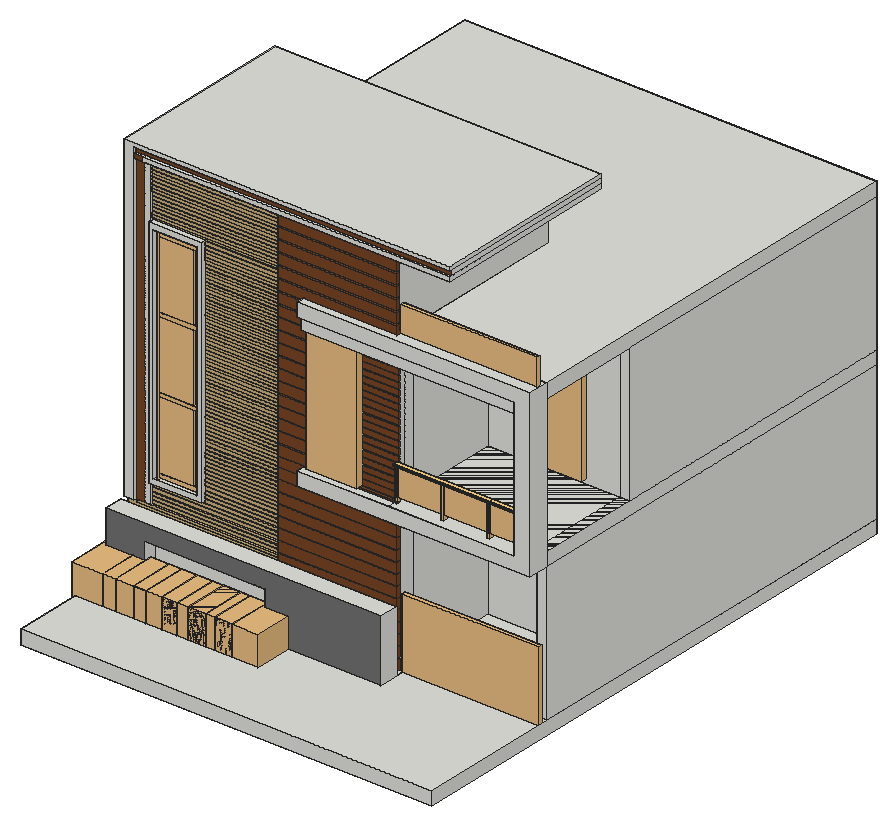
# SketchUp Ruby script. Lengths in inches.
U = 1.inch
M = Sketchup.active_model
def pt(a) = Geom::Point3d.new(a.map { |v| v * U })
def face(e, loops, mat)
  f = e.add_face(loops[0].map { |a| pt(a) })
  loops[1..].each { |l| e.add_face(l.map { |a| pt(a) }).erase! }
  f.material = f.back_material = mat if mat
  f
end
# faces: each face lists its corners as indices into pts; further lists are holes
def faces(e, pts, list, mat = nil) = list.each { |f| face(e, (f[0].is_a?(Array) ? f : [f]).map { |l| l.map { |i| pts[i] } }, mat) }
# xy, xz, yz: faces in a plane at the given z, y or x. An outline is a flat list of corners, or four numbers for a rectangle; further outlines are holes
def ring(l) = l.size == 4 ? [[l[0], l[1]], [l[2], l[1]], [l[2], l[3]], [l[0], l[3]]] : l.each_slice(2).to_a
def flat(e, list, mat, &to3) = list.each { |f| face(e, (f[0].is_a?(Array) ? f : [f]).map { |l| ring(l).map { |u, v| to3.(u, v) } }, mat) }
def xy(e, z, list, mat = nil) = flat(e, list, mat) { |x, y| [x, y, z] }
def xz(e, y, list, mat = nil) = flat(e, list, mat) { |x, z| [x, y, z] }
def yz(e, x, list, mat = nil) = flat(e, list, mat) { |y, z| [x, y, z] }
def lines(e, pts, list) = list.each { |a, b| e.add_line(pt(pts[a]), pt(pts[b])) }
# prism: a flat outline (further loops are holes) pulled along v
def prism(e, loops, v, mat = nil)
  f = face(e, loops, mat); d = Geom::Vector3d.new(v.map { |x| x * U })
  f.pushpull(f.normal.samedirection?(d) ? d.length : -d.length)
end
def box(e, o, s, mat = nil) = prism(e, [[o, [o[0] + s[0], o[1], o[2]], [o[0] + s[0], o[1] + s[1], o[2]], [o[0], o[1] + s[1], o[2]]]], [0, 0, s[2]], mat)
def at(x, y, z, deg = 0) = Geom::Transformation.translation(pt([x, y, z])) * Geom::Transformation.rotation(ORIGIN, Z_AXIS, deg.degrees)
def axes(o, x, y, z) = Geom::Transformation.new([*x, 0, *y, 0, *z, 0, *pt(o).to_a, 1])
def part(name) = M.definitions.add(name)
# library, detail: a bought-in or finely detailed component or shape, given as its bounding box
def library(name, o, s) = part(name).tap { |d| box(d.entities, o, s) }
def detail(e, o, s) = box(e.add_group.entities, o, s)
def put(e, d, t, mat = nil) = e.add_instance(d, t).tap { |i| i.material = mat if mat }
def group(e, t, mat = nil) = e.add_group.tap { |g| g.transformation = t; g.material = mat if mat }.entities
root = M.entities
M.materials.add("4wer gsdf uhghh1").color = [251, 209, 129]
M.materials.add("[0128_White]").color = [255, 255, 255]
M.materials.add("[0130_Gainsboro]").color = [220, 220, 220]
M.materials.add("[Color M05]").color = [114, 114, 114]
M.materials.add("[Wood Floor Light]").color = [204, 176, 127]
M.materials.add("[Wood Veneer 01]").color = [120, 70, 37]
c1 = library("CNC CUTTING TEXTURE",[0,0,-0.79],[85.98,295.47,0.79])
c2 = library("Untitled",[0,0,0],[36,4.39,84])
c3 = library("GATE DESIGN",[0,0,0],[157.48,1.97,82.05])
c4 = library("Raiing",[0,0,0],[2.36,157.48,43.31])
c5 = library("Line03",[-161.9,-1.5,-0.01],[5.61,3,76.05])
c6 = library("Rectangle2",[-158.32,-0.85,10.07],[105.83,1.72,65.72])
c7 = part("Rectangle3")
prism(c7.entities,[[[162.42,-2.78,77.23],[162.42,-2.8125,75.23],[162.42,2.82,75.23],[162.42,2.79,77.23],[162.42,2.57,77.68],[162.42,2.18,77.99],[162.42,1.69,78.1],[162.42,-1.68,78.1],[162.42,-2.17,77.99],[162.42,-2.5625,77.68]]],[-327.5,0,0],"4wer gsdf uhghh1")
c8 = part("skp26F")
put(c8.entities,c5,at(0,0,0))
put(c8.entities,c6,at(0,0,0))
put(c8.entities,c7,at(0,0,0))
put(c8.entities,c5,at(105.79,0,0))
put(c8.entities,c6,at(105.79,0,0))
put(c8.entities,c6,at(211.06,0,0))
put(c8.entities,c5,at(211.06,0,0))
put(c8.entities,c5,at(316.15,0,0))
c9 = part("Railing1")
put(c9.entities,c8,at(161.9,1.5,0.01))
c10 = part("plafonjera 30x30")
g1 = group(c10.entities,at(0,49.12,61.9),"[0128_White]")
xy(g1,-1.18,[[[0,-11.8125,11.8125,0],[0.79,-11.02,11.02,-0.79]]],"[0130_Gainsboro]")
xy(g1,-0.98,[[0.79,-11.02,11.02,-0.79]],"[0128_White]")
xy(g1,0,[[0,-11.8125,11.8125,0]],"[0130_Gainsboro]")
xz(g1,-11.8125,[[0,-1.18,11.8125,0]],"[0130_Gainsboro]")
xz(g1,-11.02,[[0.79,-1.18,11.02,-0.98]],"[0130_Gainsboro]")
xz(g1,-0.79,[[0.79,-1.18,11.02,-0.98]],"[0130_Gainsboro]")
xz(g1,0,[[0,-1.18,11.8125,0]],"[0130_Gainsboro]")
yz(g1,0,[[-11.8125,-1.18,0,0]],"[0130_Gainsboro]")
yz(g1,0.79,[[-11.02,-1.18,-0.79,-0.98]],"[0130_Gainsboro]")
yz(g1,11.02,[[-11.02,-1.18,-0.79,-0.98]],"[0130_Gainsboro]")
yz(g1,11.8125,[[-11.8125,-1.18,0,0]],"[0130_Gainsboro]")
c11 = library("planta",[-33.71,-17.92,-17.375],[61.06,56.98,83.04])
c12 = part("Group\#3")
box(c12.entities,[0,-0.9375,0],[32.21,0.9375,4.8125])
c13 = part("Group\#6")
box(c13.entities,[0,-3.3125,0],[104.3,3.3125,9.03])
c14 = part("Group\#5")
box(c14.entities,[78.86,-3.3125,0],[25.44,3.3125,9.03])
c15 = part("Group\#8")
box(c15.entities,[0,-1.625,0],[111.71,1.625,2.46])
c16 = part("Group\#14")
box(c16.entities,[108.55,-1.625,58.72],[65.17,1.625,2.46])
xy(root,-12,[[2.57,92.9375,2.57,125.4375,158.82,125.4375,158.82,117.5,243.57,117.5,243.57,92.9375]])
xy(root,-2.01,[[36.8125,92.9375,141.8125,104.3125]])
xy(root,0,[[2.57,109.79,243.57,117.5],[[158.82,117.5,238.63,117.5,238.63,215.88,353.57,215.88,353.57,125.4375,362.57,125.4375,362.57,485.4375,2.57,485.4375,2.57,125.4375,158.82,125.4375],[11.57,134.4375,11.57,476.4375,353.57,476.4375,353.57,224.88,229.63,224.88,229.63,134.4375]],[238.63,125.4375,353.57,134.4375],[11.57,134.4375,229.63,134.4375,229.63,224.88,353.57,224.88,353.57,476.4375,11.57,476.4375],[238.63,134.4375,353.57,215.88]])
xy(root,39.99,[[36.8125,92.9375,141.8125,104.3125]])
xy(root,54.0625,[[2.57,92.9375,243.57,109.79]])
xy(root,54.8125,[[2.57,113.25,11.57,117.5],[11.57,115.3125,18.82,117.5],[18.82,115.3125,24.75,117.5]])
xy(root,73.23,[[24.75,112.3125,71.07,117.5]])
xy(root,77.43,[[28.95,112.3125,66.875,117.5]])
xy(root,120,[[158.82,107.25,238.63,117.5],[238.63,107.25,362.57,125.4375],[158.82,117.5,238.63,125.4375],[[2.57,125.4375,238.63,125.4375,238.63,215.88,353.57,215.88,353.57,125.4375,362.57,125.4375,362.57,485.4375,2.57,485.4375],[11.57,134.4375,11.57,476.4375,353.57,476.4375,353.57,224.88,229.63,224.88,229.63,134.4375]]])
xy(root,132,[[158.82,107.25,238.63,107.25,238.63,119.75,206.42,119.75,206.42,117.5,158.82,117.5],[238.63,107.25,348.21,125.4375],[158.82,117.5,206.42,125.4375],[206.42,119.75,238.63,125.4375],[[2.57,125.4375,238.63,125.4375,238.63,215.88,362.57,215.88,362.57,485.4375,2.57,485.4375],[11.57,134.4375,11.57,476.4375,353.57,476.4375,353.57,224.88,229.63,224.88,229.63,134.4375]],
  [238.63,125.4375,362.57,125.4375,362.57,215.88,353.57,215.88,353.57,134.4375,238.63,134.4375],[11.57,134.4375,229.63,134.4375,229.63,224.88,353.57,224.88,353.57,476.4375,11.57,476.4375],[238.63,134.4375,353.57,215.88]])
xy(root,240.0625,[[158.82,111.375,158.82,117.5,206.42,117.5,206.42,119.75,238.63,119.75,238.63,125.4375,348.21,125.4375,348.21,111.375],[206.42,119.75,238.63,125.4375],[238.63,125.4375,348.21,134.4375]])
xy(root,252,[[158.82,107.25,348.21,111.375],[158.82,111.375,348.21,125.4375],[158.82,125.4375,348.21,125.4375,348.21,134.4375,238.63,134.4375,238.63,215.88,362.57,215.88,362.57,485.4375,2.57,485.4375,2.57,278.5625,11.57,278.5625,11.57,476.4375,353.57,476.4375,353.57,224.88,229.63,224.88,229.63,134.4375,158.82,134.4375],[2.57,125.4375,158.82,125.4375,158.82,134.4375,11.57,134.4375,11.57,278.5625,2.57,278.5625],[11.57,134.4375,158.82,278.5625]])
xy(root,264,[[158.82,107.25,362.57,107.25,362.57,125.4375,240.76,125.4375,240.76,117.5,158.82,117.5],[158.82,117.5,240.76,125.4375],[158.82,125.4375,240.76,278.5625]])
xy(root,272.98,[[28.95,112.3125,66.875,117.5]])
xy(root,277.17,[[24.75,112.3125,71.07,117.5]])
xy(root,322.4375,[[11.57,113.25,19.41,115.3125],[19.41,113.25,19.41,115.3125,24.75,115.3125,24.75,117.5,287.13,117.5,287.13,113.25],[11.57,117.5,18.82,125.4375],[18.82,117.5,24.75,278.5625],[24.75,117.5,240.76,278.5625],
  [240.76,117.5,287.13,278.5625],[11.57,125.4375,18.82,278.5625]])
xy(root,326.28,[[11.57,113.25,11.57,115.3125,18.82,115.3125,19.41,113.25],[19.41,113.25,18.82,115.3125,287.13,115.3125,287.13,113.25],[24.75,115.3125,287.13,278.5625]])
xy(root,330.84,[[11.57,113.25,18.82,115.3125],[18.82,113.25,287.13,115.3125],[11.57,115.3125,18.82,125.4375],[18.82,115.3125,287.13,278.5625],[11.57,125.4375,18.82,278.5625]])
xy(root,334.25,[[2.57,113.25,287.13,278.5625]])
xz(root,92.9375,[[[2.57,-12,243.57,54.0625],[36.8125,-2.01,141.8125,39.99]]],"[Color M05]")
xz(root,104.3125,[[36.8125,-2.01,141.8125,39.99]])
xz(root,107.25,[[158.82,120,362.57,120,362.57,264,158.82,264,158.82,252,348.21,252,348.21,132,158.82,132]])
xz(root,109.79,[[2.57,0,243.57,54.0625]])
xz(root,111.375,[[158.82,240.0625,348.21,252]])
xz(root,112.3125,[[[24.75,73.23,71.07,277.17],[28.95,77.43,66.875,272.98]]])
xz(root,113.25,[[2.57,54.8125,11.57,54.8125,11.57,330.84,287.13,330.84,287.13,334.25,2.57,334.25],[19.41,322.4375,287.13,326.28]])
xz(root,113.25,[[11.57,322.4375,19.41,326.28]],"[Wood Veneer 01]")
xz(root,115.3125,[[18.82,54.8125,24.75,322.4375],[11.57,322.4375,24.75,326.28]])
xz(root,115.3125,[[11.57,54.8125,18.82,322.4375],[11.57,326.28,18.82,330.84],[18.82,326.28,287.13,330.84]],"[Wood Veneer 01]")
xz(root,117.5,[[158.82,-12,243.57,0],[136.46,0,238.63,0,238.63,120,158.82,120,158.82,132,206.42,132,206.42,240.0625,158.82,240.0625,158.82,264,240.76,264,240.76,313.41,136.46,313.41],[11.57,54.8125,18.82,322.4375],[18.82,54.8125,24.75,322.4375],[28.95,77.43,66.875,272.98]])
xz(root,117.5,[[2.57,0,136.46,0,136.46,319.98,24.75,319.98,24.75,277.17,71.07,277.17,71.07,73.23,24.75,73.23,24.75,54.8125,2.57,54.8125]],"[Wood Floor Light]")
xz(root,119.75,[[206.42,132,238.63,235.25]],"[Wood Veneer 01]")
xz(root,125.4375,[[2.57,-12,158.82,0],[2.57,0,158.82,120],[353.57,0,362.57,120],[2.57,120,158.82,132],[158.82,120,362.57,132],
  [2.57,132,158.82,252],[348.21,132,348.21,252,158.82,252,158.82,264,362.57,264,362.57,132],[206.42,132,238.63,240.0625],[11.57,322.4375,18.82,330.84]])
xz(root,134.4375,[[11.57,0,229.63,120],[11.57,132,229.63,252],[238.63,240.0625,348.21,252]])
xz(root,215.88,[[238.63,0,353.57,120],[238.63,132,353.57,252],[353.57,132,362.57,252]])
xz(root,224.88,[[229.63,0,353.57,120],[229.63,132,353.57,252]])
xz(root,278.5625,[[2.57,252,158.82,252,158.82,264,240.76,264,240.76,322.4375,11.57,322.4375,11.57,330.84,287.13,330.84,287.13,334.25,2.57,334.25],[18.82,322.4375,18.82,330.84,287.13,330.84,287.13,326.28,24.75,326.28,24.75,322.4375],[24.75,322.4375,287.13,326.28]])
xz(root,476.4375,[[11.57,0,353.57,120],[11.57,132,353.57,252]])
xz(root,485.4375,[[2.57,0,362.57,120],[2.57,132,362.57,252]])
yz(root,2.57,[[92.9375,-12,92.9375,54.0625,109.79,54.0625,109.79,0,117.5,0,117.5,54.8125,113.25,54.8125,113.25,334.25,278.5625,334.25,278.5625,252,125.4375,252,125.4375,-12],[125.4375,0,485.4375,120],[125.4375,132,485.4375,252]])
yz(root,11.57,[[134.4375,0,476.4375,120],[113.25,54.8125,115.3125,322.4375],[115.3125,54.8125,115.3125,330.84,125.4375,330.84,125.4375,322.4375,117.5,322.4375,117.5,54.8125],[134.4375,132,476.4375,252],[113.25,322.4375,115.3125,326.28],
  [125.4375,322.4375,278.5625,330.84],[113.25,326.28,115.3125,330.84]])
yz(root,18.82,[[125.4375,322.4375,278.5625,330.84]])
yz(root,24.75,[[115.3125,54.8125,117.5,73.23],[112.3125,73.23,115.3125,277.17],[115.3125,73.23,117.5,277.17],[115.3125,277.17,117.5,322.4375],[115.3125,322.4375,278.5625,326.28]])
yz(root,28.95,[[112.3125,77.43,117.5,272.98]])
yz(root,36.8125,[[92.9375,-2.01,104.3125,39.99]])
yz(root,66.875,[[112.3125,77.43,117.5,272.98]])
yz(root,71.07,[[112.3125,73.23,117.5,277.17]])
yz(root,141.8125,[[92.9375,-2.01,104.3125,39.99]])
yz(root,158.82,[[117.5,-12,125.4375,0],[107.25,120,117.5,132],[117.5,120,125.4375,132],[111.375,240.0625,117.5,252],[117.5,240.0625,125.4375,252],
  [107.25,252,117.5,264],[117.5,252,125.4375,264],[125.4375,252,278.5625,264]])
yz(root,206.42,[[117.5,132,119.75,240.0625],[119.75,132,125.4375,240.0625]])
yz(root,229.63,[[134.4375,0,224.88,120],[134.4375,132,224.88,252]])
yz(root,238.63,[[117.5,0,134.4375,120],[134.4375,0,215.88,120],[119.75,132,125.4375,240.0625],[125.4375,132,134.4375,240.0625],[134.4375,132,215.88,252]])
yz(root,240.76,[[117.5,264,278.5625,322.4375]])
yz(root,243.57,[[92.9375,-12,117.5,-12,117.5,0,109.79,0,109.79,54.0625,92.9375,54.0625]])
yz(root,287.13,[[113.25,322.4375,278.5625,326.28],[115.3125,326.28,278.5625,330.84],[113.25,330.84,278.5625,334.25]])
yz(root,348.21,[[107.25,132,107.25,252,111.375,252,111.375,240.0625,125.4375,240.0625,125.4375,132],[111.375,240.0625,125.4375,252],[125.4375,240.0625,134.4375,252]])
yz(root,353.57,[[125.4375,0,215.88,120],[224.88,0,476.4375,120],[224.88,132,476.4375,252]])
yz(root,362.57,[[125.4375,0,485.4375,120],[107.25,120,125.4375,264],[215.88,132,485.4375,252]])
put(root,c1,axes([161.91,121.89,132],[0.51768,0,0],[0,0,0.36573],[0,11.28983,0]))
put(root,c2,at(288.11,211.49,135.42))
put(root,c2,at(288.11,211.49,4.48))
put(root,c3,axes([243.57,116.18,0],[0.7556,0,0],[0,1.67,0],[0,0,0.75]))
put(root,c4,axes([240.76,119.86,258.57],[0,-1,0],[0.76,0,0],[0,0,0.66]))
put(root,c9,axes([238.79,114.1875,132.875],[0.38166,0,0],[0,1,0],[0,0,0.37]))
put(root,c10,at(264.84,88.8125,259.79))
put(root,c10,at(264.84,126.125,259.79))
put(root,c10,at(264.84,163.1875,259.79))
put(root,c10,at(264.84,197.8125,259.79))
put(root,c9,axes([66.67,114.1875,79.33],[0,0,0.5971],[0,1,0],[-0.4588,0,0]))
put(root,c11,axes([20.57,72.33,-7.52],[0.6248,0,0],[0,0.68,0],[0,0,0.50364]))
put(root,c11,axes([47.38,72.33,-7.52],[0.6248,0,0],[0,0.68,0],[0,0,0.50364]))
put(root,c11,axes([74.51,72.33,-7.52],[0.6248,0,0],[0,0.68,0],[0,0,0.50364]))
put(root,c11,axes([99.2,72.33,-7.52],[0.6248,0,0],[0,0.68,0],[0,0,0.50364]))
put(root,c11,axes([122.32,72.33,-7.52],[0.6248,0,0],[0,0.68,0],[0,0,0.50364]))
put(root,c11,axes([145.32,72.33,-7.52],[0.6248,0,0],[0,0.68,0],[0,0,0.50364]))
g2 = group(root,at(2.57,485.4375,-12))
box(g2,[0,-485.4375,0],[360,485.4375,12])
g3 = group(root,at(2.57,485.4375,120))
box(g3,[0,-360,0],[360,360,12])
g4 = group(root,at(2.57,485.4375,252))
box(g4,[0,-360,0],[360,360,12])
put(root,c12,at(206.42,119.75,235.25),"[Wood Veneer 01]")
put(root,c12,at(206.42,119.75,229.75),"[Wood Veneer 01]")
put(root,c12,at(206.42,119.75,224.375),"[Wood Veneer 01]")
put(root,c12,at(206.42,119.75,218.6875),"[Wood Veneer 01]")
put(root,c12,at(206.42,119.75,213.125),"[Wood Veneer 01]")
put(root,c12,at(206.42,119.75,207.375),"[Wood Veneer 01]")
put(root,c12,at(206.42,119.75,201.8125),"[Wood Veneer 01]")
put(root,c12,at(206.42,119.75,196.125),"[Wood Veneer 01]")
put(root,c12,at(206.42,119.75,190.3125),"[Wood Veneer 01]")
put(root,c12,at(206.42,119.75,184.1875),"[Wood Veneer 01]")
put(root,c12,at(206.42,119.75,178.5),"[Wood Veneer 01]")
put(root,c12,at(206.42,119.75,172.75),"[Wood Veneer 01]")
put(root,c12,at(206.42,119.75,167),"[Wood Veneer 01]")
put(root,c12,at(206.42,119.75,161.0625),"[Wood Veneer 01]")
put(root,c12,at(206.42,119.75,155),"[Wood Veneer 01]")
put(root,c12,at(206.42,119.75,149.4375),"[Wood Veneer 01]")
put(root,c12,at(206.42,119.75,143.5625),"[Wood Veneer 01]")
put(root,c12,at(206.42,119.75,137.8125),"[Wood Veneer 01]")
put(root,c12,at(206.42,119.75,132.3125),"[Wood Veneer 01]")
put(root,c13,at(136.46,117.5,313.41),"[Wood Veneer 01]")
put(root,c13,at(136.46,117.5,302.91),"[Wood Veneer 01]")
put(root,c13,at(136.46,117.5,292.84),"[Wood Veneer 01]")
put(root,c13,at(136.46,117.5,282.59),"[Wood Veneer 01]")
put(root,c13,at(136.46,117.5,272.53),"[Wood Veneer 01]")
put(root,c13,at(136.46,117.5,262.28),"[Wood Veneer 01]")
put(root,c13,at(136.46,117.5,252.22),"[Wood Veneer 01]")
put(root,c13,at(136.46,117.5,242.16),"[Wood Veneer 01]")
put(root,c14,at(57.6,117.5,232.09),"[Wood Veneer 01]")
put(root,c14,at(57.6,117.5,222.09),"[Wood Veneer 01]")
put(root,c14,at(57.6,117.5,212.09),"[Wood Veneer 01]")
put(root,c14,at(57.6,117.5,202.09),"[Wood Veneer 01]")
put(root,c14,at(57.6,117.5,192.22),"[Wood Veneer 01]")
put(root,c14,at(57.6,117.5,182.34),"[Wood Veneer 01]")
put(root,c14,at(57.6,117.5,172.47),"[Wood Veneer 01]")
put(root,c14,at(57.6,117.5,162.78),"[Wood Veneer 01]")
put(root,c14,at(57.6,117.5,152.97),"[Wood Veneer 01]")
put(root,c14,at(57.6,117.5,143.16),"[Wood Veneer 01]")
put(root,c14,at(57.6,117.5,132.59),"[Wood Veneer 01]")
put(root,c13,at(136.46,117.5,0),"[Wood Veneer 01]")
put(root,c13,at(136.46,117.5,9.9375),"[Wood Veneer 01]")
put(root,c13,at(136.46,117.5,19.5),"[Wood Veneer 01]")
put(root,c13,at(136.46,117.5,28.9375),"[Wood Veneer 01]")
put(root,c13,at(136.46,117.5,38.5),"[Wood Veneer 01]")
put(root,c13,at(136.46,117.5,47.9375),"[Wood Veneer 01]")
put(root,c13,at(136.46,117.5,57.5),"[Wood Veneer 01]")
put(root,c13,at(136.46,117.5,67.0625),"[Wood Veneer 01]")
put(root,c13,at(136.46,117.5,76.625),"[Wood Veneer 01]")
put(root,c13,at(136.46,117.5,86.125),"[Wood Veneer 01]")
put(root,c13,at(136.46,117.5,95.625),"[Wood Veneer 01]")
put(root,c13,at(136.46,117.5,105.25),"[Wood Veneer 01]")
put(root,c13,at(136.46,117.5,114.8125),"[Wood Veneer 01]")
put(root,c13,at(136.46,117.5,123.84),"[Wood Veneer 01]")
put(root,c15,at(24.75,117.5,319.98),"[Wood Floor Light]")
put(root,c15,at(24.75,117.5,317.16),"[Wood Floor Light]")
put(root,c15,at(24.75,117.5,314.35),"[Wood Floor Light]")
put(root,c15,at(24.75,117.5,311.54),"[Wood Floor Light]")
put(root,c15,at(24.75,117.5,308.6),"[Wood Floor Light]")
put(root,c15,at(24.75,117.5,305.66),"[Wood Floor Light]")
put(root,c15,at(24.75,117.5,302.73),"[Wood Floor Light]")
put(root,c15,at(24.75,117.5,299.79),"[Wood Floor Light]")
put(root,c15,at(24.75,117.5,296.91),"[Wood Floor Light]")
put(root,c15,at(24.75,117.5,293.91),"[Wood Floor Light]")
put(root,c15,at(24.75,117.5,290.98),"[Wood Floor Light]")
put(root,c15,at(24.75,117.5,288.1),"[Wood Floor Light]")
put(root,c15,at(24.75,117.5,285.16),"[Wood Floor Light]")
put(root,c15,at(24.75,117.5,282.35),"[Wood Floor Light]")
put(root,c15,at(24.75,117.5,279.54),"[Wood Floor Light]")
put(root,c16,at(-37.25,117.5,215.84),"[Wood Floor Light]")
put(root,c16,at(-37.25,117.5,212.02),"[Wood Floor Light]")
put(root,c16,at(-37.25,117.5,209.21),"[Wood Floor Light]")
put(root,c16,at(-37.25,117.5,206.4),"[Wood Floor Light]")
put(root,c16,at(-37.25,117.5,203.59),"[Wood Floor Light]")
put(root,c16,at(-37.48,117.5,200.89),"[Wood Floor Light]")
put(root,c16,at(-37.48,117.5,198.21),"[Wood Floor Light]")
put(root,c16,at(-37.48,117.5,195.27),"[Wood Floor Light]")
put(root,c16,at(-37.48,117.5,192.64),"[Wood Floor Light]")
put(root,c16,at(-37.48,117.5,189.89),"[Wood Floor Light]")
put(root,c16,at(-37.48,117.5,187.07),"[Wood Floor Light]")
put(root,c16,at(-37.48,117.5,184.32),"[Wood Floor Light]")
put(root,c16,at(-37.48,117.5,181.5),"[Wood Floor Light]")
put(root,c16,at(-37.48,117.5,178.93),"[Wood Floor Light]")
put(root,c16,at(-37.48,117.5,176.24),"[Wood Floor Light]")
put(root,c16,at(-37.48,117.5,173.68),"[Wood Floor Light]")
put(root,c16,at(-37.48,117.5,170.99),"[Wood Floor Light]")
put(root,c16,at(-37.48,117.5,168.3),"[Wood Floor Light]")
put(root,c16,at(-37.48,117.5,165.68),"[Wood Floor Light]")
put(root,c16,at(-37.48,117.5,163.11),"[Wood Floor Light]")
put(root,c16,at(-37.48,117.5,160.55),"[Wood Floor Light]")
put(root,c16,at(-37.48,117.5,158),"[Wood Floor Light]")
put(root,c16,at(-37.48,117.5,155.4375),"[Wood Floor Light]")
put(root,c16,at(-37.48,117.5,152.75),"[Wood Floor Light]")
put(root,c16,at(-37.48,117.5,150.125),"[Wood Floor Light]")
put(root,c16,at(-37.48,117.5,147.4375),"[Wood Floor Light]")
put(root,c16,at(-37.48,117.5,144.5625),"[Wood Floor Light]")
put(root,c16,at(-37.48,117.5,141.8125),"[Wood Floor Light]")
put(root,c16,at(-37.48,117.5,138.9375),"[Wood Floor Light]")
put(root,c16,at(-37.48,117.5,136.25),"[Wood Floor Light]")
put(root,c16,at(-37.48,117.5,133.625),"[Wood Floor Light]")
put(root,c16,at(-37.48,117.5,130.8125),"[Wood Floor Light]")
put(root,c16,at(-37.48,117.5,127.96),"[Wood Floor Light]")
put(root,c16,at(-37.48,117.5,125.21),"[Wood Floor Light]")
put(root,c16,at(-37.48,117.5,122.54),"[Wood Floor Light]")
put(root,c16,at(-37.48,117.5,119.97),"[Wood Floor Light]")
put(root,c16,at(-37.48,117.5,117.16),"[Wood Floor Light]")
put(root,c16,at(-37.48,117.5,114.35),"[Wood Floor Light]")
put(root,c16,at(-37.48,117.5,111.54),"[Wood Floor Light]")
put(root,c16,at(-37.48,117.5,108.72),"[Wood Floor Light]")
put(root,c16,at(-37.48,117.5,105.91),"[Wood Floor Light]")
put(root,c16,at(-37.48,117.5,103.1),"[Wood Floor Light]")
put(root,c16,at(-37.48,117.5,100.29),"[Wood Floor Light]")
put(root,c16,at(-37.48,117.5,97.47),"[Wood Floor Light]")
put(root,c16,at(-37.48,117.5,94.66),"[Wood Floor Light]")
put(root,c16,at(-37.48,117.5,91.85),"[Wood Floor Light]")
put(root,c16,at(-37.48,117.5,89.04),"[Wood Floor Light]")
put(root,c16,at(-37.48,117.5,86.04),"[Wood Floor Light]")
put(root,c16,at(-37.48,117.5,83.04),"[Wood Floor Light]")
put(root,c16,at(-37.48,117.5,80.04),"[Wood Floor Light]")
put(root,c16,at(-37.48,117.5,77.04),"[Wood Floor Light]")
put(root,c16,at(-37.48,117.5,74.04),"[Wood Floor Light]")
put(root,c16,at(-37.48,117.5,71.04),"[Wood Floor Light]")
put(root,c16,at(-37.48,117.5,68.04),"[Wood Floor Light]")
put(root,c16,at(-37.48,117.5,65.04),"[Wood Floor Light]")
put(root,c16,at(-37.48,117.5,62.04),"[Wood Floor Light]")
put(root,c16,at(-37.48,117.5,59.04),"[Wood Floor Light]")
put(root,c16,at(-37.48,117.5,55.85),"[Wood Floor Light]")
put(root,c16,at(-37.48,117.5,52.66),"[Wood Floor Light]")
put(root,c16,at(-37.48,117.5,49.47),"[Wood Floor Light]")
put(root,c16,at(-37.48,117.5,46.29),"[Wood Floor Light]")
put(root,c16,at(-37.48,117.5,43.1),"[Wood Floor Light]")
put(root,c16,at(-37.48,117.5,39.91),"[Wood Floor Light]")
put(root,c16,at(-37.48,117.5,36.72),"[Wood Floor Light]")
put(root,c16,at(-37.48,117.5,33.54),"[Wood Floor Light]")
put(root,c16,at(-37.48,117.5,30.35),"[Wood Floor Light]")
put(root,c16,at(-37.48,117.5,27.16),"[Wood Floor Light]")
put(root,c16,at(-37.48,117.5,23.79),"[Wood Floor Light]")
put(root,c16,at(-37.48,117.5,20.41),"[Wood Floor Light]")
put(root,c16,at(-37.48,117.5,17.04),"[Wood Floor Light]")
put(root,c16,at(-37.48,117.5,13.66),"[Wood Floor Light]")
g5 = group(root,at(-37.48,117.5,10.29),"[Wood Floor Light]")
box(g5,[49.05,-1.625,58.72],[124.67,1.625,2.46])
g6 = group(root,at(-37.48,117.5,6.91),"[Wood Floor Light]")
box(g6,[49.05,-1.625,58.72],[124.67,1.625,2.46])
g7 = group(root,at(-37.48,117.5,3.54),"[Wood Floor Light]")
box(g7,[49.05,-1.625,58.72],[124.67,1.625,2.46])
g8 = group(root,at(-37.48,117.5,0.16),"[Wood Floor Light]")
box(g8,[49.05,-1.625,58.72],[124.67,1.625,2.46])
g9 = group(root,at(-37.48,117.5,-3.21),"[Wood Floor Light]")
box(g9,[49.05,-1.625,58.72],[124.67,1.625,2.46])
g10 = group(root,at(-37.48,117.5,-6.59),"[Wood Floor Light]")
box(g10,[49.05,-1.625,58.72],[124.67,1.625,2.46])
